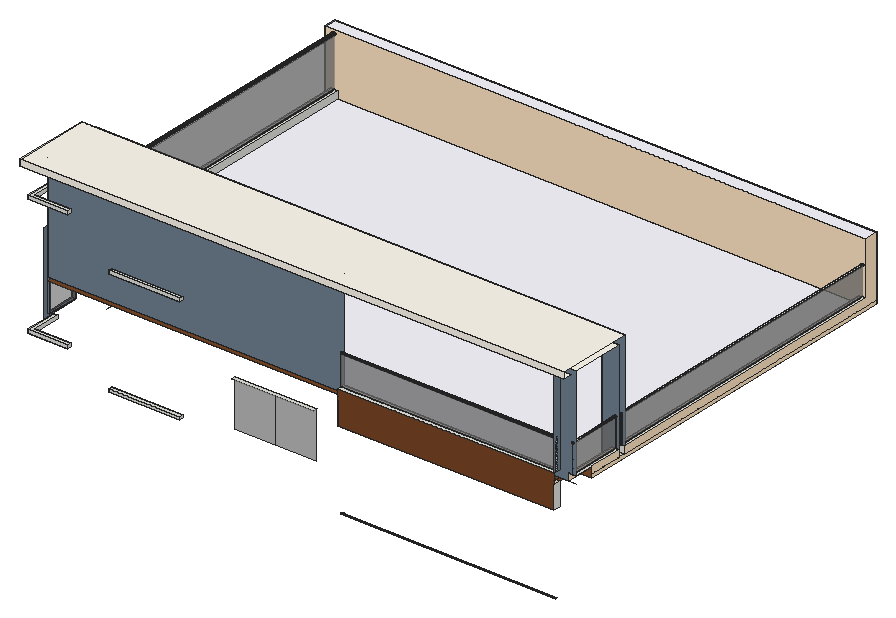
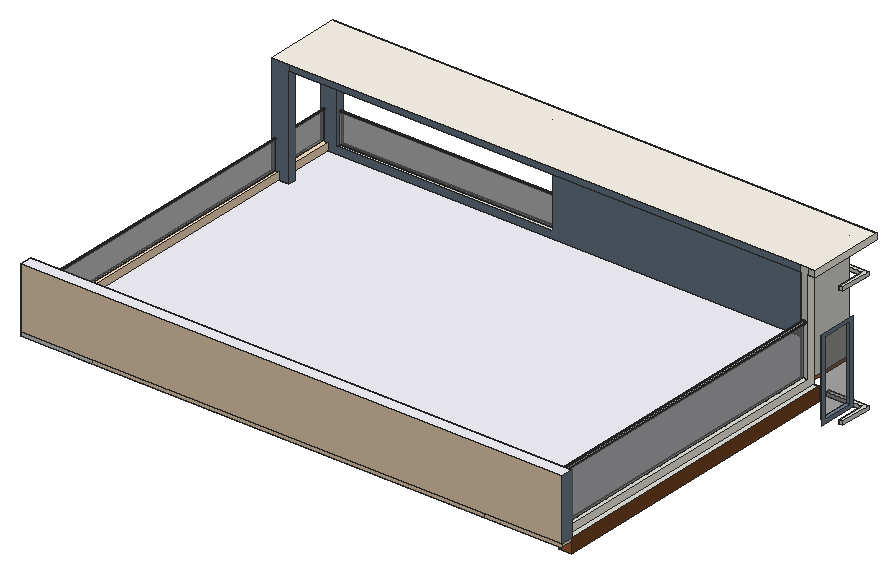
# SketchUp Ruby script. Lengths in inches.
U = 1.inch
M = Sketchup.active_model
def pt(a) = Geom::Point3d.new(a.map { |v| v * U })
def face(e, loops, mat)
  f = e.add_face(loops[0].map { |a| pt(a) })
  loops[1..].each { |l| e.add_face(l.map { |a| pt(a) }).erase! }
  f.material = f.back_material = mat if mat
  f
end
# faces: each face lists its corners as indices into pts; further lists are holes
def faces(e, pts, list, mat = nil) = list.each { |f| face(e, (f[0].is_a?(Array) ? f : [f]).map { |l| l.map { |i| pts[i] } }, mat) }
# xy, xz, yz: faces in a plane at the given z, y or x. An outline is a flat list of corners, or four numbers for a rectangle; further outlines are holes
def ring(l) = l.size == 4 ? [[l[0], l[1]], [l[2], l[1]], [l[2], l[3]], [l[0], l[3]]] : l.each_slice(2).to_a
def flat(e, list, mat, &to3) = list.each { |f| face(e, (f[0].is_a?(Array) ? f : [f]).map { |l| ring(l).map { |u, v| to3.(u, v) } }, mat) }
def xy(e, z, list, mat = nil) = flat(e, list, mat) { |x, y| [x, y, z] }
def xz(e, y, list, mat = nil) = flat(e, list, mat) { |x, z| [x, y, z] }
def yz(e, x, list, mat = nil) = flat(e, list, mat) { |y, z| [x, y, z] }
def lines(e, pts, list) = list.each { |a, b| e.add_line(pt(pts[a]), pt(pts[b])) }
# prism: a flat outline (further loops are holes) pulled along v
def prism(e, loops, v, mat = nil)
  f = face(e, loops, mat); d = Geom::Vector3d.new(v.map { |x| x * U })
  f.pushpull(f.normal.samedirection?(d) ? d.length : -d.length)
end
def box(e, o, s, mat = nil) = prism(e, [[o, [o[0] + s[0], o[1], o[2]], [o[0] + s[0], o[1] + s[1], o[2]], [o[0], o[1] + s[1], o[2]]]], [0, 0, s[2]], mat)
def at(x, y, z, deg = 0) = Geom::Transformation.translation(pt([x, y, z])) * Geom::Transformation.rotation(ORIGIN, Z_AXIS, deg.degrees)
def axes(o, x, y, z) = Geom::Transformation.new([*x, 0, *y, 0, *z, 0, *pt(o).to_a, 1])
def part(name) = M.definitions.add(name)
# library, detail: a bought-in or finely detailed component or shape, given as its bounding box
def library(name, o, s) = part(name).tap { |d| box(d.entities, o, s) }
def detail(e, o, s) = box(e.add_group.entities, o, s)
def put(e, d, t, mat = nil) = e.add_instance(d, t).tap { |i| i.material = mat if mat }
def group(e, t, mat = nil) = e.add_group.tap { |g| g.transformation = t; g.material = mat if mat }.entities
root = M.entities
M.materials.add("[0008_LavenderBlush]").color = [255, 240, 245]
M.materials.add("[0012_Bisque]").color = [255, 228, 196]
M.materials.add("[0021_DarkRed]").color = [76, 0, 0]
M.materials.add("[0052_FloralWhite]").color = [255, 250, 240]
M.materials.add("[0111_SlateGray]").color = [112, 128, 144]
M.materials.add("[0117_GhostWhite]").color = [248, 248, 255]
M.materials.add("[Translucent Glass Gray]").color = [84, 84, 84]
M.materials["[Translucent Glass Gray]"].alpha = 0.5
M.materials.add("[Translucent Glass Gray]1").color = [128, 128, 128]
M.materials["[Translucent Glass Gray]1"].alpha = 0.5
M.materials.add("[Translucent Resin Crush Gray]").color = [153, 153, 153]
M.materials["[Translucent Resin Crush Gray]"].alpha = 0.8
M.materials.add("[Wood Veneer 01]").color = [120, 70, 37]
box(root,[282.03,96,1731.25],[240.38,12,10.38])
box(root,[282.03,96,2087.13],[240.38,12,10.37])
prism(root,[[[24,204,2216.39],[24,108,2216.39],[144,108,2216.39],[144,96,2216.39],[12,96,2216.39],[12,204,2216.39]]],[0,0,12])
xy(root,1644.0625,[[1061.52,588,1118.46,589.5]])
xy(root,1803.1875,[[1061.52,588,1118.46,589.5]])
xy(root,1803.1875,[[1263.97,588,1442.1,589.5]],"[0021_DarkRed]")
xy(root,1813.2,[[12,96,24,108],[24,96,144,108],[12,108,24,204]])
xy(root,1825.2,[[12,96,144,96,144,108,24,108,24,204,12,204]])
xy(root,1851.3125,[[24,158.55,36,264.68]],"[0111_SlateGray]")
xy(root,1891.5,[[1044,108,1767.4375,132]],"[Wood Veneer 01]")
xy(root,1916.49,[[695.08,96,971.45,108]])
xy(root,1932,[[6,312,48,1350]],"[Wood Veneer 01]")
xy(root,1968,[[153.42,451.1875,150.3125,451.6,147.42,452.8,144.93,454.7,143.02,457.1875,141.83,460.08,141.42,463.1875,141.83,466.29,143.02,469.1875,144.93,471.67,147.42,473.58,150.3125,474.78,153.42,475.1875,156.52,474.78,159.42,473.58,161.9,471.67,163.81,469.1875,165.01,466.29,165.42,463.1875,165.01,460.08,163.81,457.1875,161.9,454.7,159.42,452.8,156.52,451.6],[264,588,1584,1392],[153.42,595.1875,150.3125,595.6,147.42,596.8,144.93,598.7,143.02,601.1875,141.83,604.08,141.42,607.1875,141.83,610.29,143.02,613.1875,144.93,615.67,147.42,617.58,150.3125,618.78,153.42,619.1875,156.52,618.78,159.42,617.58,161.9,615.67,163.81,613.1875,165.01,610.29,165.42,607.1875,165.01,604.08,163.81,601.1875,161.9,598.7,159.42,596.8,156.52,595.6],[153.42,739.1875,150.3125,739.6,147.42,740.8,144.93,742.7,143.02,745.1875,141.83,748.08,141.42,751.1875,141.83,754.29,143.02,757.1875,144.93,759.67,147.42,761.58,150.3125,762.78,153.42,763.1875,156.52,762.78,159.42,761.58,161.9,759.67,163.81,757.1875,165.01,754.29,165.42,751.1875,165.01,748.08,163.81,745.1875,161.9,742.7,159.42,740.8,156.52,739.6],[153.42,883.1875,150.3125,883.6,147.42,884.8,144.93,886.7,143.02,889.1875,141.83,892.08,141.42,895.1875,141.83,898.29,143.02,901.1875,144.93,903.67,147.42,905.58,150.3125,906.78,153.42,907.1875,156.52,906.78,159.42,905.58,161.9,903.67,163.81,901.1875,165.01,898.29,165.42,895.1875,165.01,892.08,163.81,889.1875,161.9,886.7,159.42,884.8,156.52,883.6],
  [153.42,1027.1875,150.3125,1027.6,147.42,1028.8,144.93,1030.7,143.02,1033.1875,141.83,1036.08,141.42,1039.1875,141.83,1042.29,143.02,1045.1875,144.93,1047.67,147.42,1049.58,150.3125,1050.78,153.42,1051.1875,156.52,1050.78,159.42,1049.58,161.9,1047.67,163.81,1045.1875,165.01,1042.29,165.42,1039.1875,165.01,1036.08,163.81,1033.1875,161.9,1030.7,159.42,1028.8,156.52,1027.6],[153.42,1171.1875,150.3125,1171.6,147.42,1172.8,144.93,1174.7,143.02,1177.1875,141.83,1180.08,141.42,1183.1875,141.83,1186.29,143.02,1189.1875,144.93,1191.67,147.42,1193.58,150.3125,1194.78,153.42,1195.1875,156.52,1194.78,159.42,1193.58,161.9,1191.67,163.81,1189.1875,165.01,1186.29,165.42,1183.1875,165.01,1180.08,163.81,1177.1875,161.9,1174.7,159.42,1172.8,156.52,1171.6]])
xy(root,1968,[[1034.09,362.21,1027.82,362.35,1021.81,364.09,1016.45,367.34,1012.11,371.86,1009.09,377.35,1007.6,383.4375,1007.73,389.7,1009.48,395.72,1012.72,401.08,1017.25,405.41,1022.74,408.43,1028.82,409.92,1035.08,409.79,1041.1,408.05,1046.46,404.8,1050.8,400.28,1053.8125,394.79,1055.31,388.7,1055.18,382.4375,1053.43,376.42,1050.18,371.0625,1045.66,366.73,1040.17,363.71],[1310.09,362.21,1303.82,362.35,1297.81,364.09,1292.45,367.34,1288.11,371.86,1285.09,377.35,1283.6,383.4375,1283.73,389.7,1285.48,395.72,1288.72,401.08,1293.25,405.41,1298.74,408.43,1304.82,409.92,1311.08,409.79,1317.1,408.05,1322.46,404.8,1326.8,400.28,1329.8125,394.79,1331.31,388.7,1331.18,382.4375,1329.43,376.42,1326.18,371.0625,1321.66,366.73,1316.17,363.71],[1586.09,362.21,1579.82,362.35,1573.81,364.09,1568.45,367.34,1564.11,371.86,1561.09,377.35,1559.6,383.4375,1559.73,389.7,1561.48,395.72,1564.72,401.08,1569.25,405.41,1574.74,408.43,1580.82,409.92,1587.08,409.79,1593.1,408.05,1598.46,404.8,1602.8,400.28,1605.8125,394.79,1607.31,388.7,1607.18,382.4375,1605.43,376.42,1602.18,371.0625,1597.66,366.73,1592.17,363.71],[1721.5,663.5,1715.29,664.3125,1709.5,666.71,1704.53,670.53,1700.72,675.5,1698.32,681.28,1697.5,687.5,1698.32,693.71,1700.72,699.5,1704.53,704.47,1709.5,708.28,1715.29,710.68,1721.5,711.5,1727.71,710.68,1733.5,708.28,1738.47,704.47,1742.29,699.5,1744.68,693.71,1745.5,687.5,1744.68,681.28,1742.29,675.5,1738.47,670.53,1733.5,666.71,1727.71,664.3125],[1721.5,987.5,1715.29,988.3125,1709.5,990.71,1704.53,994.53,1700.72,999.5,1698.32,1005.28,1697.5,1011.5,1698.32,1017.71,1700.72,1023.5,1704.53,1028.47,1709.5,1032.28,1715.29,1034.68,1721.5,1035.5,1727.71,1034.68,1733.5,1032.28,1738.47,1028.47,1742.29,1023.5,1744.68,1017.71,1745.5,1011.5,1744.68,1005.28,1742.29,999.5,1738.47,994.53,1733.5,990.71,1727.71,988.3125]],"[0008_LavenderBlush]")
xy(root,1968,[[[48,132,48,1392,264,1392,264,588,1584,588,1584,1392,1745,1392,1745,1284,1824,1284,1824,199.52,1767.4375,199.52,1767.4375,132],[1034.09,362.21,1040.17,363.71,1045.66,366.73,1050.18,371.0625,1053.43,376.42,1055.18,382.4375,1055.31,388.7,1053.8125,394.79,1050.8,400.28,1046.46,404.8,1041.1,408.05,1035.08,409.79,1028.82,409.92,1022.74,408.43,1017.25,405.41,1012.72,401.08,1009.48,395.72,1007.73,389.7,1007.6,383.4375,1009.09,377.35,1012.11,371.86,1016.45,367.34,1021.81,364.09,1027.82,362.35],[1310.09,362.21,1316.17,363.71,1321.66,366.73,1326.18,371.0625,1329.43,376.42,1331.18,382.4375,1331.31,388.7,1329.8125,394.79,1326.8,400.28,1322.46,404.8,1317.1,408.05,1311.08,409.79,1304.82,409.92,1298.74,408.43,1293.25,405.41,1288.72,401.08,1285.48,395.72,1283.73,389.7,1283.6,383.4375,1285.09,377.35,1288.11,371.86,1292.45,367.34,1297.81,364.09,1303.82,362.35],[1586.09,362.21,1592.17,363.71,1597.66,366.73,1602.18,371.0625,1605.43,376.42,1607.18,382.4375,1607.31,388.7,1605.8125,394.79,1602.8,400.28,1598.46,404.8,1593.1,408.05,1587.08,409.79,1580.82,409.92,1574.74,408.43,1569.25,405.41,1564.72,401.08,1561.48,395.72,1559.73,389.7,1559.6,383.4375,1561.09,377.35,1564.11,371.86,1568.45,367.34,1573.81,364.09,1579.82,362.35],[1721.5,663.5,1727.71,664.3125,1733.5,666.71,1738.47,670.53,1742.29,675.5,1744.68,681.28,1745.5,687.5,1744.68,693.71,1742.29,699.5,1738.47,704.47,1733.5,708.28,1727.71,710.68,1721.5,711.5,1715.29,710.68,1709.5,708.28,1704.53,704.47,1700.72,699.5,1698.32,693.71,1697.5,687.5,1698.32,681.28,1700.72,675.5,1704.53,670.53,1709.5,666.71,1715.29,664.3125],[1721.5,987.5,1727.71,988.3125,1733.5,990.71,1738.47,994.53,1742.29,999.5,1744.68,1005.28,1745.5,1011.5,1744.68,1017.71,1742.29,1023.5,1738.47,1028.47,1733.5,1032.28,1727.71,1034.68,1721.5,1035.5,1715.29,1034.68,1709.5,1032.28,1704.53,1028.47,1700.72,1023.5,1698.32,1017.71,1697.5,1011.5,1698.32,1005.28,1700.72,999.5,1704.53,994.53,1709.5,990.71,1715.29,988.3125],[153.42,1171.1875,156.52,1171.6,159.42,1172.8,161.9,1174.7,163.81,1177.1875,165.01,1180.08,165.42,1183.1875,165.01,1186.29,163.81,1189.1875,161.9,1191.67,159.42,1193.58,156.52,1194.78,153.42,1195.1875,150.3125,1194.78,147.42,1193.58,144.93,1191.67,143.02,1189.1875,141.83,1186.29,141.42,1183.1875,141.83,1180.08,143.02,1177.1875,144.93,1174.7,147.42,1172.8,150.3125,1171.6],[153.42,1027.1875,156.52,1027.6,159.42,1028.8,161.9,1030.7,163.81,1033.1875,165.01,1036.08,165.42,1039.1875,165.01,1042.29,163.81,1045.1875,161.9,1047.67,159.42,1049.58,156.52,1050.78,153.42,1051.1875,150.3125,1050.78,147.42,1049.58,144.93,1047.67,143.02,1045.1875,141.83,1042.29,141.42,1039.1875,141.83,1036.08,143.02,1033.1875,144.93,1030.7,147.42,1028.8,150.3125,1027.6],[153.42,883.1875,156.52,883.6,159.42,884.8,161.9,886.7,163.81,889.1875,165.01,892.08,165.42,895.1875,165.01,898.29,163.81,901.1875,161.9,903.67,159.42,905.58,156.52,906.78,153.42,907.1875,150.3125,906.78,147.42,905.58,144.93,903.67,143.02,901.1875,141.83,898.29,141.42,895.1875,141.83,892.08,143.02,889.1875,144.93,886.7,147.42,884.8,150.3125,883.6],[153.42,739.1875,156.52,739.6,159.42,740.8,161.9,742.7,163.81,745.1875,165.01,748.08,165.42,751.1875,165.01,754.29,163.81,757.1875,161.9,759.67,159.42,761.58,156.52,762.78,153.42,763.1875,150.3125,762.78,147.42,761.58,144.93,759.67,143.02,757.1875,141.83,754.29,141.42,751.1875,141.83,748.08,143.02,745.1875,144.93,742.7,147.42,740.8,150.3125,739.6],[153.42,595.1875,156.52,595.6,159.42,596.8,161.9,598.7,163.81,601.1875,165.01,604.08,165.42,607.1875,165.01,610.29,163.81,613.1875,161.9,615.67,159.42,617.58,156.52,618.78,153.42,619.1875,150.3125,618.78,147.42,617.58,144.93,615.67,143.02,613.1875,141.83,610.29,141.42,607.1875,141.83,604.08,143.02,601.1875,144.93,598.7,147.42,596.8,150.3125,595.6],[153.42,451.1875,156.52,451.6,159.42,452.8,161.9,454.7,163.81,457.1875,165.01,460.08,165.42,463.1875,165.01,466.29,163.81,469.1875,161.9,471.67,159.42,473.58,156.52,474.78,153.42,475.1875,150.3125,474.78,147.42,473.58,144.93,471.67,143.02,469.1875,141.83,466.29,141.42,463.1875,141.83,460.08,143.02,457.1875,144.93,454.7,147.42,452.8,150.3125,451.6]]],"[Wood Veneer 01]")
xy(root,1980,[[6,312,24,1350],[24,312,48,336],[1767.4375,312,1824,336],[24,336,24,1350,6,1350,6,1392,1824,1392,1824,336,1800,336,1800,1350,48,1350,48,336]])
xy(root,1980,[[48,132,1800,132,1800,312,1767.4375,312,1767.4375,336,1800,336,1800,1350,48,1350]],"[0117_GhostWhite]")
xy(root,2004,[[1044,108,1767.4375,118.5],[1044,118.5,1767.4375,120],[1044,120,1767.4375,132],[1812,132,1813.5,312],[1813.5,132,1824,312],
  [24,336,36,1350],[36,336,38,1350],[38,336,48,1350],[1812,336,1813,1350],[1813,336,1824,1350],
  [36,1350,38,1368],[1812,1350,1813,1368]])
xy(root,2004,[[1800,132,1812,312],[1800,336,1812,1350]],"[0012_Bisque]")
xy(root,2097,[[1812,132,1813.5,312]])
xy(root,2100,[[1812,336,1813,1368]])
xy(root,2101.3125,[[24,158.55,36,264.68]],"[0111_SlateGray]")
xy(root,2103,[[1044,118.5,1767.4375,120]])
xy(root,2166,[[36,336,38,1368]])
xy(root,2184,[[6,1350,1824,1392]],"[0117_GhostWhite]")
xy(root,2319.6,[[534,96,1044,108]])
xy(root,2319.6,[[0,78,0,336,24,336,24,108,534,108,534,96,1044,96,1044,132,48,132,48,336,1767.4375,336,1767.4375,312,1824,312,1824,132,1767.4375,132,1767.4375,108,1824,108,1824,78]],"[0052_FloralWhite]")
xy(root,2340,[[0,78,1824,336]],"[0052_FloralWhite]")
xz(root,78,[[0,2319.6,1824,2340]],"[0052_FloralWhite]")
xz(root,96,[[12,1813.2,144,1825.2]])
xz(root,108,[[24,1813.2,144,1825.2]])
xz(root,108,[[695.08,1757.62,833.27,1916.49],[833.27,1757.62,971.45,1916.49]],"[Translucent Resin Crush Gray]")
xz(root,108,[[1044,1891.5,1767.4375,2004]],"[Wood Veneer 01]")
xz(root,118.5,[[1044,2004,1767.4375,2103]],"[Translucent Glass Gray]1")
xz(root,120,[[1044,2103,1767.4375,2106]])
xz(root,120,[[1044,2004,1767.4375,2103]],"[Translucent Glass Gray]1")
xz(root,132,[[1812,2004,1813.5,2097],[1812,2097,1812.78,2097.1,1813.5,2097.4,1814.12,2097.88,1814.6,2098.5,1814.9,2099.22,1815,2100,1814.9,2100.78,1814.6,2101.5,1814.12,2102.12,1813.5,2102.6,1812.78,2102.9,1812,2103,1811.22,2102.9,1810.5,2102.6,1809.88,2102.12,1809.4,2101.5,1809.1,2100.78,1809,2100,1809.1,2099.22,1809.4,2098.5,1809.88,2097.88,1810.5,2097.4,1811.22,2097.1]])
xz(root,132,[[1044,1891.5,1767.4375,1968]],"[0012_Bisque]")
xz(root,132,[[[48,1980,48,2319.6,1044,2319.6,1044,2004,1767.4375,2004,1767.4375,2319.6,1824,2319.6,1824,2004,1800,2004,1800,1980],[1812,2097,1812.78,2097.1,1813.5,2097.4,1814.12,2097.88,1814.6,2098.5,1814.9,2099.22,1815,2100,1814.9,2100.78,1814.6,2101.5,1814.12,2102.12,1813.5,2102.6,1812.78,2102.9,1812,2103,1811.22,2102.9,1810.5,2102.6,1809.88,2102.12,1809.4,2101.5,1809.1,2100.78,1809,2100,1809.1,2099.22,1809.4,2098.5,1809.88,2097.88,1810.5,2097.4,1811.22,2097.1]]],"[0111_SlateGray]")
xz(root,158.55,[[24,1851.3125,36,2101.3125]],"[0111_SlateGray]")
xz(root,204,[[12,1813.2,24,1825.2]])
xz(root,264.68,[[24,1851.3125,36,2101.3125]],"[0111_SlateGray]")
xz(root,312,[[24,1932,48,1968],[1800,1980,1824,2004],[1812,2004,1813.5,2097]])
xz(root,312,[[[1767.4375,1980,1800,1980,1800,2004,1824,2004,1824,2319.6,1767.4375,2319.6],[1812,2097,1811.22,2097.1,1810.5,2097.4,1809.88,2097.88,1809.4,2098.5,1809.1,2099.22,1809,2100,1809.1,2100.78,1809.4,2101.5,1809.88,2102.12,1810.5,2102.6,1811.22,2102.9,1812,2103,1812.78,2102.9,1813.5,2102.6,1814.12,2102.12,1814.6,2101.5,1814.9,2100.78,1815,2100,1814.9,2099.22,1814.6,2098.5,1814.12,2097.88,1813.5,2097.4,1812.78,2097.1]]],"[0111_SlateGray]")
xz(root,312,[[6,1932,24,1980]],"[Wood Veneer 01]")
xz(root,336,[[1800,1980,1824,2004],[[24,2004,48,2340],[36,2166,37.55,2166.2,39,2166.8,40.24,2167.76,41.2,2169,41.8,2170.45,42,2172,41.8,2173.55,41.2,2175,40.24,2176.24,39,2177.2,37.55,2177.8,36,2178,34.45,2177.8,33,2177.2,31.76,2176.24,30.8,2175,30.2,2173.55,30,2172,30.2,2170.45,30.8,2169,31.76,2167.76,33,2166.8,34.45,2166.2]],[36,2004,38,2166],[1812,2004,1813,2004,1813,2097.01,1812.08,2097.01,1812.05,2097,1812,2097.01],[1812.05,2097,1812.08,2097.01,1812,2097.01],
  [1812,2097.01,1812.08,2097.01,1812.82,2097.11,1813,2097.19,1813,2100,1812,2100],[1812.08,2097.01,1813,2097.01,1813,2097.19,1812.82,2097.11],[36,2166,37.55,2166.2,39,2166.8,40.24,2167.76,41.2,2169,41.8,2170.45,42,2172,41.8,2173.55,41.2,2175,40.24,2176.24,39,2177.2,37.55,2177.8,36,2178,34.45,2177.8,33,2177.2,31.76,2176.24,30.8,2175,30.2,2173.55,30,2172,30.2,2170.45,30.8,2169,31.76,2167.76,33,2166.8,34.45,2166.2],[0,2319.6,24,2340]])
xz(root,336,[[[1767.4375,1980,1767.4375,2340,1824,2340,1824,2004,1800,2004,1800,1980],[1812.05,2097,1812.08,2097.01,1812.82,2097.11,1813,2097.19,1813.54,2097.42,1814.15,2097.91,1814.62,2098.54,1814.91,2099.27,1815,2100.05,1814.89,2100.82,1814.58,2101.54,1814.09,2102.15,1813.46,2102.62,1812.73,2102.91,1811.95,2103,1811.18,2102.89,1810.46,2102.58,1809.85,2102.09,1809.38,2101.46,1809.09,2100.73,1809,2099.95,1809.11,2099.18,1809.42,2098.46,1809.91,2097.85,1810.54,2097.38,1811.27,2097.09,1812,2097.01]],[48,2319.6,1767.4375,2340]],"[0111_SlateGray]")
xz(root,588,[[[1053.52,1636.0625,1126.46,1811.1875],[1061.52,1644.0625,1118.46,1803.1875]]],"[0021_DarkRed]")
xz(root,589.5,[[1061.52,1644.0625,1118.46,1803.1875]],"[Translucent Glass Gray]")
xz(root,1350,[[[6,1980,24,1980,24,2004,48,2004,48,1980,1800,1980,1800,2004,1824,2004,1824,2184,6,2184],[36,2166,34.45,2166.2,33,2166.8,31.76,2167.76,30.8,2169,30.2,2170.45,30,2172,30.2,2173.55,30.8,2175,31.76,2176.24,33,2177.2,34.45,2177.8,36,2178,37.55,2177.8,39,2177.2,40.24,2176.24,41.2,2175,41.8,2173.55,42,2172,41.8,2170.45,41.2,2169,40.24,2167.76,39,2166.8,37.55,2166.2],[1812.05,2097,1812,2097.01,1811.27,2097.09,1810.54,2097.38,1809.91,2097.85,1809.42,2098.46,1809.11,2099.18,1809,2099.95,1809.09,2100.73,1809.38,2101.46,1809.85,2102.09,1810.46,2102.58,1811.18,2102.89,1811.95,2103,1812.73,2102.91,1813.46,2102.62,1814.09,2102.15,1814.58,2101.54,1814.89,2100.82,1815,2100.05,1814.91,2099.27,1814.62,2098.54,1814.15,2097.91,1813.54,2097.42,1813,2097.19,1812.82,2097.11,1812.08,2097.01]]],"[0012_Bisque]")
xz(root,1368,[[36,2004,38,2166],[1812,2004,1812,2097.01,1812.05,2097,1812.08,2097.01,1813,2097.01,1813,2004],[1812.05,2097,1812,2097.01,1812.08,2097.01],[1812,2097.01,1811.27,2097.09,1810.54,2097.38,1809.91,2097.85,1809.42,2098.46,1809.11,2099.18,1809,2099.95,1809.09,2100.73,1809.38,2101.46,1809.85,2102.09,1810.46,2102.58,1811.18,2102.89,1811.95,2103,1812.73,2102.91,1813.46,2102.62,1814.09,2102.15,1814.58,2101.54,1814.89,2100.82,1815,2100.05,1814.91,2099.27,1814.62,2098.54,1814.15,2097.91,1813.54,2097.42,1813,2097.19,1813,2100,1812,2100],[1812,2097.01,1812,2100,1813,2100,1813,2097.19,1812.82,2097.11,1812.08,2097.01],
  [1812.08,2097.01,1812.82,2097.11,1813,2097.19,1813,2097.01]])
xz(root,1392,[[1584,1968,1824,1980]])
xz(root,1392,[[6,1968,264,1980],[264,1968,1584,1980],[6,1980,1824,2184]],"[0012_Bisque]")
yz(root,0,[[78,2319.6,336,2340]],"[0052_FloralWhite]")
yz(root,6,[[1350,1980,1392,2184]],"[0111_SlateGray]")
yz(root,6,[[312,1932,1350,1980]],"[Wood Veneer 01]")
yz(root,12,[[96,1813.2,204,1825.2]])
yz(root,24,[[108,1813.2,204,1825.2]])
yz(root,24,[[312,1980,312,2319.6,336,2319.6,336,2004,1350,2004,1350,1980]],"[0052_FloralWhite]")
yz(root,24,[[[146.55,1839.3125,276.68,2113.3125],[158.55,1851.3125,264.68,2101.3125]]],"[0111_SlateGray]")
yz(root,36,[[336,2166,1368,2172]])
yz(root,36,[[158.55,1851.3125,264.68,2101.3125]],"[Translucent Glass Gray]")
yz(root,36,[[336,2004,1368,2166]],"[Translucent Glass Gray]1")
yz(root,38,[[336,2004,1368,2166]],"[Translucent Glass Gray]1")
yz(root,48,[[132,1980,336,2319.6],[336,1980,1350,2004]])
yz(root,48,[[312,1932,1350,1968]],"[0012_Bisque]")
yz(root,144,[[96,1813.2,108,1825.2]])
yz(root,1044,[[108,1891.5,132,1968],[118.5,2004,120,2103]])
yz(root,1061.52,[[588,1644.0625,589.5,1803.1875]])
yz(root,1118.46,[[588,1644.0625,589.5,1803.1875]])
yz(root,1767.4375,[[108,1891.5,132,1968],[118.5,2004,120,2103],[120,2103,120.3125,2103.02,120.625,2103.07,120.93,2103.15,121.22,2103.26,121.5,2103.4,121.76,2103.57,122.01,2103.77,122.23,2103.99,122.43,2104.24,122.6,2104.5,122.74,2104.78,122.85,2105.07,122.93,2105.375,122.98,2105.6875,123,2106,122.98,2106.3125,122.93,2106.625,122.85,2106.93,122.74,2107.22,122.6,2107.5,122.43,2107.76,122.23,2108.01,122.01,2108.23,121.76,2108.43,121.5,2108.6,121.22,2108.74,120.93,2108.85,120.625,2108.93,120.3125,2108.98,120,2109,119.6875,2108.98,119.375,2108.93,119.07,2108.85,118.78,2108.74,118.5,2108.6,118.24,2108.43,117.99,2108.23,117.77,2108.01,117.57,2107.76,117.4,2107.5,117.26,2107.22,117.15,2106.93,117.07,2106.625,117.02,2106.3125,117,2106,117.02,2105.6875,117.07,2105.375,117.15,2105.07,117.26,2104.78,117.4,2104.5,117.57,2104.24,117.77,2103.99,117.99,2103.77,118.24,2103.57,118.5,2103.4,118.78,2103.26,119.07,2103.15,119.375,2103.07,119.6875,2103.02]])
yz(root,1767.4375,[[312,1980,336,2319.6],[[108,2004,132,2319.6],[120,2103,120.3125,2103.02,120.625,2103.07,120.93,2103.15,121.22,2103.26,121.5,2103.4,121.76,2103.57,122.01,2103.77,122.23,2103.99,122.43,2104.24,122.6,2104.5,122.74,2104.78,122.85,2105.07,122.93,2105.375,122.98,2105.6875,123,2106,122.98,2106.3125,122.93,2106.625,122.85,2106.93,122.74,2107.22,122.6,2107.5,122.43,2107.76,122.23,2108.01,122.01,2108.23,121.76,2108.43,121.5,2108.6,121.22,2108.74,120.93,2108.85,120.625,2108.93,120.3125,2108.98,120,2109,119.6875,2108.98,119.375,2108.93,119.07,2108.85,118.78,2108.74,118.5,2108.6,118.24,2108.43,117.99,2108.23,117.77,2108.01,117.57,2107.76,117.4,2107.5,117.26,2107.22,117.15,2106.93,117.07,2106.625,117.02,2106.3125,117,2106,117.02,2105.6875,117.07,2105.375,117.15,2105.07,117.26,2104.78,117.4,2104.5,117.57,2104.24,117.77,2103.99,117.99,2103.77,118.24,2103.57,118.5,2103.4,118.78,2103.26,119.07,2103.15,119.375,2103.07,119.6875,2103.02]]],"[0111_SlateGray]")
yz(root,1800,[[132,1980,312,2004],[336,1980,1350,2004]],"[0012_Bisque]")
yz(root,1812,[[132,2097,312,2100]])
yz(root,1812,[[132,2004,312,2097],[336,2004,1368,2100]],"[Translucent Glass Gray]1")
yz(root,1813,[[336,2004,1368,2100]],"[Translucent Glass Gray]1")
yz(root,1813.5,[[132,2004,312,2097]],"[Translucent Glass Gray]1")
yz(root,1824,[[199.52,1968,1392,1980],[199.52,1980,312,2004],[336,1980,1392,1980,1392,2184,1350,2184,1350,2004,336,2004]],"[0012_Bisque]")
p = [[1767.4375,117.4,1621.5],[1767.4375,117.88,1622.12],[1044,117.88,1622.12],[1044,117.4,1621.5],[1767.4375,122.12,1622.12],[1767.4375,122.6,1621.5],
  [1044,122.6,1621.5],[1044,122.12,1622.12],[1767.4375,118.5,1622.6],[1044,118.5,1622.6],[1767.4375,121.5,1622.6],[1044,121.5,1622.6],
  [1767.4375,119.22,1622.9],[1044,119.22,1622.9],[1767.4375,120.78,1622.9],[1044,120.78,1622.9],[1767.4375,120,1623],[1044,120,1623],
  [1812,132,2097],[1811.22,132,2097.1],[1811.22,312,2097.1],[1812,312,2097],[1812.78,132,2097.1],[1812.78,312,2097.1],
  [1811.27,336,2097.09],[1811.27,1350,2097.09],[1812,1350,2097.01],[1812.05,1350,2097],[1812.05,336,2097],[1812,336,2097.01],
  [1812.08,1350,2097.01],[1812.82,1350,2097.11],[1812.82,336,2097.11],[1812.08,336,2097.01],[1811.27,1368,2097.09],[1812,1368,2097.01],
  [1812.05,1368,2097],[1812.08,1368,2097.01],[1812.82,1368,2097.11],[1810.5,132,2097.4],[1810.5,312,2097.4],[1813.5,132,2097.4],
  [1813.5,312,2097.4],[1810.54,336,2097.38],[1810.54,1350,2097.38],[1813,1350,2097.19],[1813.54,1350,2097.42],[1813.54,336,2097.42],
  [1813,336,2097.19],[1810.54,1368,2097.38],[1813,1368,2097.19],[1813.54,1368,2097.42],[1809.88,132,2097.88],[1809.88,312,2097.88],
  [1814.12,132,2097.88],[1814.12,312,2097.88],[1809.91,336,2097.85],[1809.91,1350,2097.85],[1814.15,1350,2097.91],[1814.15,336,2097.91],
  [1809.91,1368,2097.85],[1814.15,1368,2097.91],[1809.42,336,2098.46],[1809.42,1350,2098.46],[1809.42,1368,2098.46],[1809.4,132,2098.5],
  [1809.4,312,2098.5],[1814.6,132,2098.5],[1814.6,312,2098.5],[1814.62,1350,2098.54],[1814.62,336,2098.54],[1814.62,1368,2098.54],
  [1809.1,132,2099.22],[1809.1,312,2099.22],[1814.9,132,2099.22],[1814.9,312,2099.22],[1809.11,336,2099.18],[1809.11,1350,2099.18],
  [1814.91,1350,2099.27],[1814.91,336,2099.27],[1809.11,1368,2099.18],[1814.91,1368,2099.27],[1809,132,2100],[1809,312,2100],
  [1815,132,2100],[1815,312,2100],[1809,336,2099.95],[1809,1350,2099.95],[1809,1368,2099.95],[1815,1350,2100.05],
  [1815,336,2100.05],[1815,1368,2100.05],[1809.1,132,2100.78],[1809.1,312,2100.78],[1814.9,132,2100.78],[1814.9,312,2100.78],
  [1809.09,336,2100.73],[1809.09,1350,2100.73],[1814.89,1350,2100.82],[1814.89,336,2100.82],[1809.09,1368,2100.73],[1814.89,1368,2100.82],
  [1809.38,336,2101.46],[1809.38,1350,2101.46],[1809.38,1368,2101.46],[1809.4,132,2101.5],[1809.4,312,2101.5],[1814.6,132,2101.5],
  [1814.6,312,2101.5],[1814.58,1350,2101.54],[1814.58,336,2101.54],[1814.58,1368,2101.54],[1809.88,132,2102.12],[1809.88,312,2102.12],
  [1814.12,132,2102.12],[1814.12,312,2102.12],[1809.85,336,2102.09],[1809.85,1350,2102.09],[1814.09,1350,2102.15],[1814.09,336,2102.15],
  [1809.85,1368,2102.09],[1814.09,1368,2102.15],[1810.5,132,2102.6],[1810.5,312,2102.6],[1813.5,132,2102.6],[1813.5,312,2102.6],
  [1810.46,336,2102.58],[1810.46,1350,2102.58],[1810.46,1368,2102.58],[1813.46,1350,2102.62],[1813.46,336,2102.62],[1813.46,1368,2102.62],
  [1811.22,132,2102.9],[1811.22,312,2102.9],[1812.78,132,2102.9],[1812.78,312,2102.9],[1811.18,336,2102.89],[1811.18,1350,2102.89],
  [1812.73,1350,2102.91],[1812.73,336,2102.91],[1811.18,1368,2102.89],[1812.73,1368,2102.91],[1812,132,2103],[1812,312,2103],
  [1811.95,336,2103],[1811.95,1350,2103],[1811.95,1368,2103],[1767.4375,119.6875,2103.02],[1767.4375,119.375,2103.07],[1044,119.375,2103.07],
  [1044,119.6875,2103.02],[1767.4375,120,2103],[1044,120,2103],[1767.4375,120.3125,2103.02],[1044,120.3125,2103.02],[1767.4375,120.625,2103.07],
  [1044,120.625,2103.07],[1767.4375,119.07,2103.15],[1767.4375,118.78,2103.26],[1044,118.78,2103.26],[1044,119.07,2103.15],[1767.4375,120.93,2103.15],
  [1044,120.93,2103.15],[1767.4375,121.22,2103.26],[1044,121.22,2103.26],[1767.4375,118.5,2103.4],[1044,118.5,2103.4],[1767.4375,121.5,2103.4],
  [1044,121.5,2103.4],[1767.4375,118.24,2103.57],[1044,118.24,2103.57],[1767.4375,121.76,2103.57],[1044,121.76,2103.57],[1767.4375,117.99,2103.77],
  [1044,117.99,2103.77],[1767.4375,122.01,2103.77],[1044,122.01,2103.77],[1767.4375,117.77,2103.99],[1044,117.77,2103.99],[1767.4375,122.23,2103.99],
  [1044,122.23,2103.99],[1767.4375,117.57,2104.24],[1044,117.57,2104.24],[1767.4375,122.43,2104.24],[1044,122.43,2104.24],[1767.4375,117.4,2104.5],
  [1044,117.4,2104.5],[1767.4375,122.6,2104.5],[1044,122.6,2104.5],[1767.4375,117.26,2104.78],[1044,117.26,2104.78],[1767.4375,122.74,2104.78],
  [1044,122.74,2104.78],[1767.4375,117.15,2105.07],[1044,117.15,2105.07],[1767.4375,122.85,2105.07],[1044,122.85,2105.07],[1767.4375,117.07,2105.375],
  [1044,117.07,2105.375],[1767.4375,122.93,2105.375],[1044,122.93,2105.375],[1767.4375,117.02,2105.6875],[1044,117.02,2105.6875],[1767.4375,122.98,2105.6875],
  [1044,122.98,2105.6875],[1767.4375,117,2106],[1044,117,2106],[1767.4375,123,2106],[1044,123,2106],[1767.4375,117.02,2106.3125],
  [1044,117.02,2106.3125],[1767.4375,122.98,2106.3125],[1044,122.98,2106.3125],[1767.4375,117.07,2106.625],[1044,117.07,2106.625],[1767.4375,122.93,2106.625],
  [1044,122.93,2106.625],[1767.4375,117.15,2106.93],[1044,117.15,2106.93],[1767.4375,122.85,2106.93],[1044,122.85,2106.93],[1767.4375,117.26,2107.22],
  [1044,117.26,2107.22],[1767.4375,122.74,2107.22],[1044,122.74,2107.22],[1767.4375,117.4,2107.5],[1044,117.4,2107.5],[1767.4375,122.6,2107.5],
  [1044,122.6,2107.5],[1767.4375,117.57,2107.76],[1044,117.57,2107.76],[1767.4375,122.43,2107.76],[1044,122.43,2107.76],[1767.4375,117.77,2108.01],
  [1044,117.77,2108.01],[1767.4375,122.23,2108.01],[1044,122.23,2108.01],[1767.4375,117.99,2108.23],[1044,117.99,2108.23],[1767.4375,122.01,2108.23],
  [1044,122.01,2108.23],[1767.4375,118.24,2108.43],[1044,118.24,2108.43],[1767.4375,121.76,2108.43],[1044,121.76,2108.43],[1767.4375,118.5,2108.6],
  [1044,118.5,2108.6],[1767.4375,121.5,2108.6],[1044,121.5,2108.6],[1767.4375,118.78,2108.74],[1044,118.78,2108.74],[1767.4375,121.22,2108.74],
  [1044,121.22,2108.74],[1767.4375,119.07,2108.85],[1044,119.07,2108.85],[1767.4375,120.93,2108.85],[1044,120.93,2108.85],[1767.4375,119.375,2108.93],
  [1044,119.375,2108.93],[1767.4375,119.6875,2108.98],[1044,119.6875,2108.98],[1767.4375,120.3125,2108.98],[1767.4375,120.625,2108.93],[1044,120.625,2108.93],
  [1044,120.3125,2108.98],[1767.4375,120,2109],[1044,120,2109],[36,336,2166],[34.45,336,2166.2],[34.45,1350,2166.2],
  [36,1350,2166],[37.55,336,2166.2],[37.55,1350,2166.2],[33,336,2166.8],[33,1350,2166.8],[39,336,2166.8],
  [39,1350,2166.8],[31.76,336,2167.76],[31.76,1350,2167.76],[40.24,336,2167.76],[40.24,1350,2167.76],[30.8,336,2169],
  [30.8,1350,2169],[41.2,336,2169],[41.2,1350,2169],[30.2,336,2170.45],[30.2,1350,2170.45],[41.8,336,2170.45],
  [41.8,1350,2170.45],[30,336,2172],[30,1350,2172],[42,336,2172],[42,1350,2172],[30.2,336,2173.55],
  [30.2,1350,2173.55],[41.8,336,2173.55],[41.8,1350,2173.55],[30.8,336,2175],[30.8,1350,2175],[41.2,336,2175],
  [41.2,1350,2175],[31.76,336,2176.24],[31.76,1350,2176.24],[40.24,336,2176.24],[40.24,1350,2176.24],[33,336,2177.2],
  [33,1350,2177.2],[39,336,2177.2],[39,1350,2177.2],[34.45,336,2177.8],[34.45,1350,2177.8],[37.55,336,2177.8],
  [37.55,1350,2177.8],[36,336,2178],[36,1350,2178],[264,132,1968],[264,108,1968],[48,1350,1968],
  [24,1350,1968],[1824,132,1980],[1800,132,1980],[1767.4375,132,1980],[1767.4375,108,1980],[48,132,2319.6],
  [48,132,2340],[1044,132,2319.6],[1044,132,2340],[1044,108,1980],[1044,132,1980]]
faces(root,p,[[0,1,2,3],[4,5,6,7],[1,8,9,2],[10,4,7,11],[8,12,13,9],[14,10,11,15],[12,16,17,13],[16,14,15,17],
  [18,19,20,21],[22,18,21,23],[24,25,26,27,28,29],[28,27,30,31,32,33],[34,35,26,25],[35,36,27,26],[36,37,30,27],[37,38,31,30],
  [19,39,40,20],[41,22,23,42],[43,44,25,24],[32,31,45,46,47,48],[49,34,25,44],[38,50,45,31],[50,51,46,45],[39,52,53,40],
  [54,41,42,55],[56,57,44,43],[47,46,58,59],[60,49,44,57],[51,61,58,46],[62,63,57,56],[64,60,57,63],[52,65,66,53],
  [67,54,55,68],[59,58,69,70],[61,71,69,58],[65,72,73,66],[74,67,68,75],[76,77,63,62],[70,69,78,79],[80,64,63,77],
  [71,81,78,69],[72,82,83,73],[84,74,75,85],[86,87,77,76],[88,80,77,87],[79,78,89,90],[81,91,89,78],[82,92,93,83],
  [94,84,85,95],[96,97,87,86],[90,89,98,99],[100,88,87,97],[91,101,98,89],[102,103,97,96],[104,100,97,103],[92,105,106,93],
  [107,94,95,108],[99,98,109,110],[101,111,109,98],[105,112,113,106],[114,107,108,115],[116,117,103,102],[110,109,118,119],[120,104,103,117],
  [111,121,118,109],[112,122,123,113],[124,114,115,125],[126,127,117,116],[128,120,117,127],[119,118,129,130],[121,131,129,118],[122,132,133,123],
  [134,124,125,135],[136,137,127,126],[130,129,138,139],[140,128,127,137],[131,141,138,129],[132,142,143,133],[142,134,135,143],[144,145,137,136],
  [139,138,145,144],[146,140,137,145],[141,146,145,138],[147,148,149,150],[151,147,150,152],[153,151,152,154],[155,153,154,156],[157,158,159,160],
  [148,157,160,149],[161,155,156,162],[163,161,162,164],[158,165,166,159],[167,163,164,168],[165,169,170,166],[171,167,168,172],[169,173,174,170],
  [175,171,172,176],[173,177,178,174],[179,175,176,180],[177,181,182,178],[183,179,180,184],[181,185,186,182],[187,183,184,188],[185,189,190,186],
  [191,187,188,192],[189,193,194,190],[195,191,192,196],[193,197,198,194],[199,195,196,200],[197,201,202,198],[203,199,200,204],[201,205,206,202],
  [207,203,204,208],[205,209,210,206],[211,207,208,212],[209,213,214,210],[215,211,212,216],[213,217,218,214],[219,215,216,220],[217,221,222,218],
  [223,219,220,224],[221,225,226,222],[227,223,224,228],[225,229,230,226],[231,227,228,232],[229,233,234,230],[235,231,232,236],[233,237,238,234],
  [239,235,236,240],[237,241,242,238],[243,239,240,244],[241,245,246,242],[247,243,244,248],[245,249,250,246],[251,247,248,252],[249,253,254,250],
  [255,251,252,256],[253,257,258,254],[257,259,260,258],[261,262,263,264],[262,255,256,263],[259,265,266,260],[265,261,264,266],[267,268,269,270],
  [271,267,270,272],[268,273,274,269],[275,271,272,276],[273,277,278,274],[279,275,276,280],[277,281,282,278],[283,279,280,284],[281,285,286,282],
  [287,283,284,288],[285,289,290,286],[291,287,288,292],[289,293,294,290],[295,291,292,296],[293,297,298,294],[299,295,296,300],[297,301,302,298],
  [303,299,300,304],[301,305,306,302],[307,303,304,308],[305,309,310,306],[311,307,308,312],[309,313,314,310],[313,311,312,314]])
lines(root,p,[[315,316],[317,318],[319,320],[321,322],[323,324],[325,326],[327,328]])
